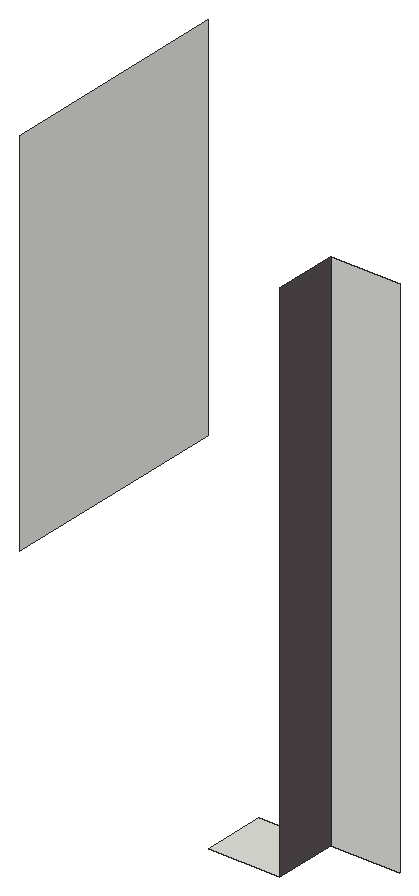
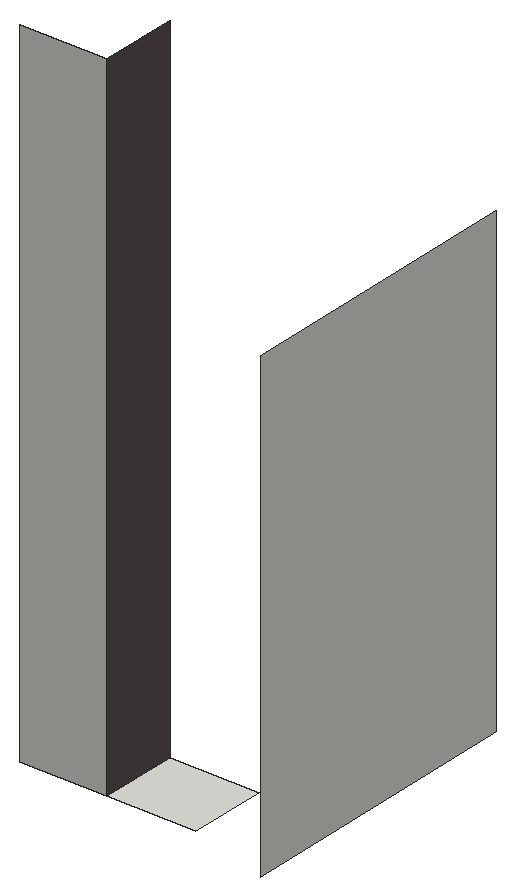
# SketchUp Ruby script. Lengths in inches.
U = 1.inch
M = Sketchup.active_model
def pt(a) = Geom::Point3d.new(a.map { |v| v * U })
def face(e, loops, mat)
  f = e.add_face(loops[0].map { |a| pt(a) })
  loops[1..].each { |l| e.add_face(l.map { |a| pt(a) }).erase! }
  f.material = f.back_material = mat if mat
  f
end
# faces: each face lists its corners as indices into pts; further lists are holes
def faces(e, pts, list, mat = nil) = list.each { |f| face(e, (f[0].is_a?(Array) ? f : [f]).map { |l| l.map { |i| pts[i] } }, mat) }
# xy, xz, yz: faces in a plane at the given z, y or x. An outline is a flat list of corners, or four numbers for a rectangle; further outlines are holes
def ring(l) = l.size == 4 ? [[l[0], l[1]], [l[2], l[1]], [l[2], l[3]], [l[0], l[3]]] : l.each_slice(2).to_a
def flat(e, list, mat, &to3) = list.each { |f| face(e, (f[0].is_a?(Array) ? f : [f]).map { |l| ring(l).map { |u, v| to3.(u, v) } }, mat) }
def xy(e, z, list, mat = nil) = flat(e, list, mat) { |x, y| [x, y, z] }
def xz(e, y, list, mat = nil) = flat(e, list, mat) { |x, z| [x, y, z] }
def yz(e, x, list, mat = nil) = flat(e, list, mat) { |y, z| [x, y, z] }
def lines(e, pts, list) = list.each { |a, b| e.add_line(pt(pts[a]), pt(pts[b])) }
# prism: a flat outline (further loops are holes) pulled along v
def prism(e, loops, v, mat = nil)
  f = face(e, loops, mat); d = Geom::Vector3d.new(v.map { |x| x * U })
  f.pushpull(f.normal.samedirection?(d) ? d.length : -d.length)
end
def box(e, o, s, mat = nil) = prism(e, [[o, [o[0] + s[0], o[1], o[2]], [o[0] + s[0], o[1] + s[1], o[2]], [o[0], o[1] + s[1], o[2]]]], [0, 0, s[2]], mat)
def at(x, y, z, deg = 0) = Geom::Transformation.translation(pt([x, y, z])) * Geom::Transformation.rotation(ORIGIN, Z_AXIS, deg.degrees)
def axes(o, x, y, z) = Geom::Transformation.new([*x, 0, *y, 0, *z, 0, *pt(o).to_a, 1])
def part(name) = M.definitions.add(name)
# library, detail: a bought-in or finely detailed component or shape, given as its bounding box
def library(name, o, s) = part(name).tap { |d| box(d.entities, o, s) }
def detail(e, o, s) = box(e.add_group.entities, o, s)
def put(e, d, t, mat = nil) = e.add_instance(d, t).tap { |i| i.material = mat if mat }
def group(e, t, mat = nil) = e.add_group.tap { |g| g.transformation = t; g.material = mat if mat }.entities
root = M.entities
M.materials.add("[Asphalt New]").color = [91, 82, 84]
xy(root,24.68,[[330.33,92.3,334.81,96.24]])
xz(root,96.24,[[334.81,24.68,339.17,57.8125]])
yz(root,315.3,[[96.24,34.41,111,57.8125]])
yz(root,334.81,[[92.3,24.68,96.24,57.8125]],"[Asphalt New]")
